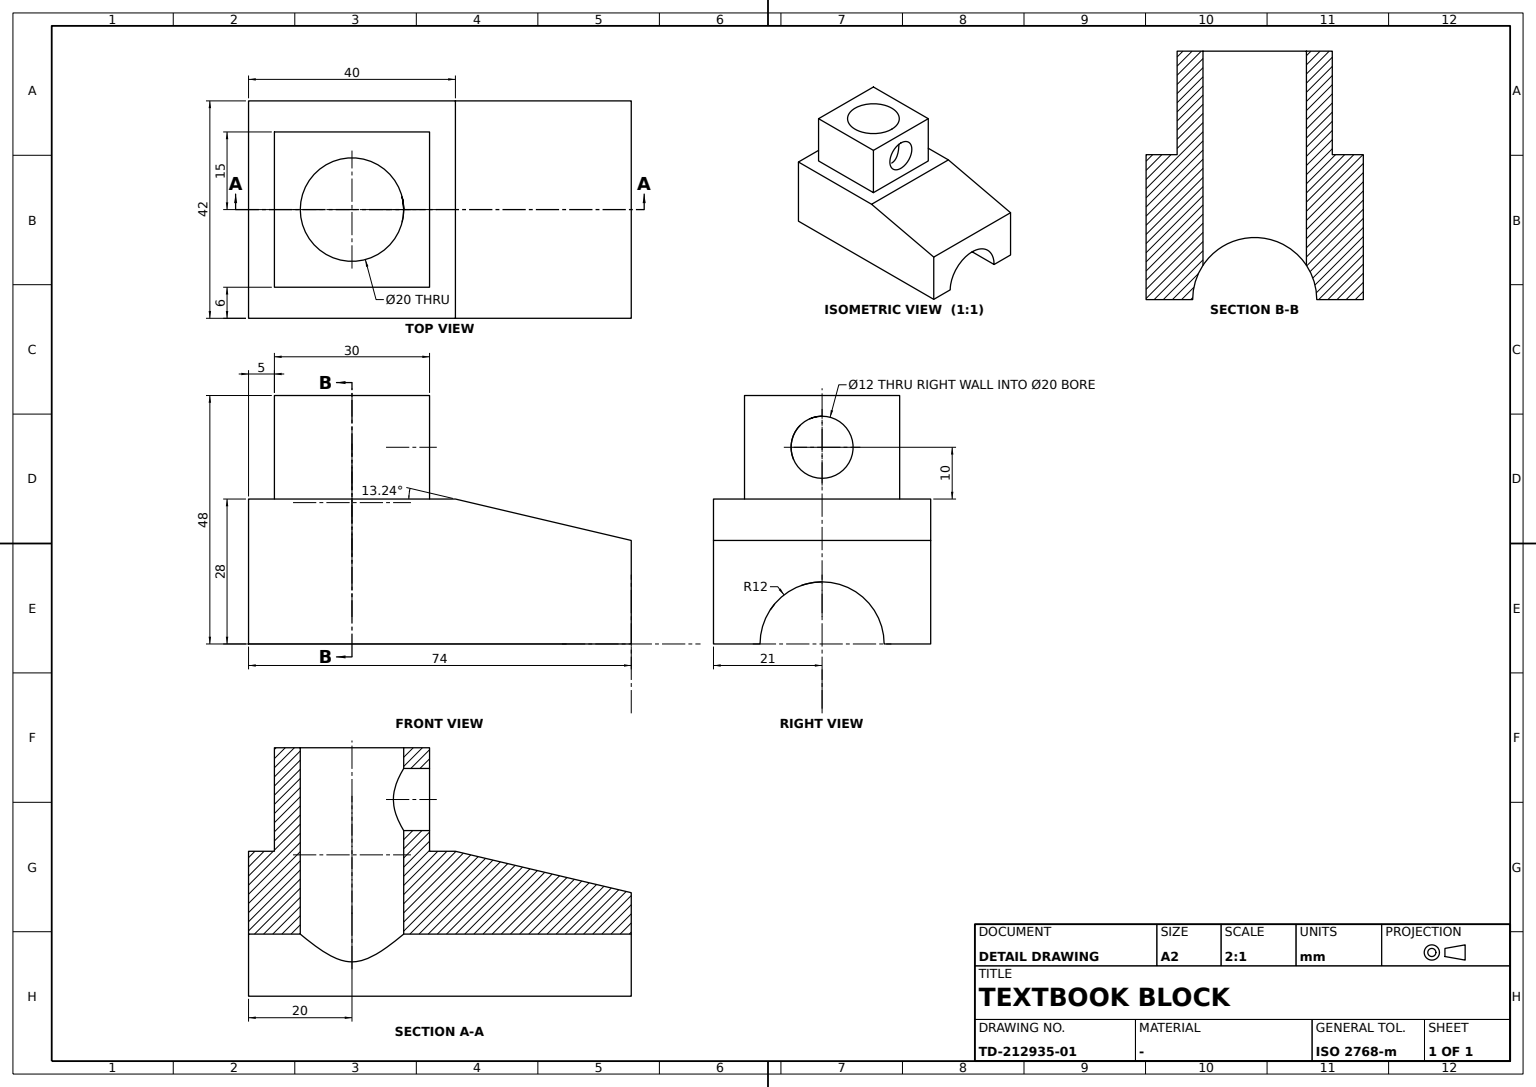
ISO-10303-21;
HEADER;
FILE_DESCRIPTION((''),'2;1');
FILE_NAME('','',(''),(''),'','','');
FILE_SCHEMA(('AUTOMOTIVE_DESIGN'));
ENDSEC;
DATA;
#1=APPLICATION_CONTEXT('');
#2=PRODUCT_CONTEXT('',#1,'mechanical');
#3=PRODUCT('','','',(#2));
#4=PRODUCT_DEFINITION_FORMATION('','',#3);
#5=PRODUCT_DEFINITION_CONTEXT('',#1,'design');
#6=PRODUCT_DEFINITION('','',#4,#5);
#7=PRODUCT_DEFINITION_SHAPE('','',#6);
#8=(LENGTH_UNIT()NAMED_UNIT(*)SI_UNIT(.MILLI.,.METRE.));
#9=(NAMED_UNIT(*)PLANE_ANGLE_UNIT()SI_UNIT($,.RADIAN.));
#10=(NAMED_UNIT(*)SI_UNIT($,.STERADIAN.)SOLID_ANGLE_UNIT());
#11=UNCERTAINTY_MEASURE_WITH_UNIT(LENGTH_MEASURE(0.005),#8,'distance_accuracy_value','');
#12=(GEOMETRIC_REPRESENTATION_CONTEXT(3)GLOBAL_UNCERTAINTY_ASSIGNED_CONTEXT((#11))GLOBAL_UNIT_ASSIGNED_CONTEXT((#8,#9,#10))REPRESENTATION_CONTEXT('',''));
#13=CARTESIAN_POINT('',(-69.,15.,48.));
#14=VERTEX_POINT('',#13);
#15=CARTESIAN_POINT('',(-39.,15.,48.));
#16=VERTEX_POINT('',#15);
#17=CARTESIAN_POINT('',(0.,15.,48.));
#18=DIRECTION('',(1.,0.,0.));
#19=VECTOR('',#18,1000.);
#20=LINE('',#17,#19);
#21=EDGE_CURVE('',#14,#16,#20,.T.);
#22=ORIENTED_EDGE('',*,*,#21,.T.);
#23=CARTESIAN_POINT('',(-39.,15.,28.));
#24=VERTEX_POINT('',#23);
#25=DIRECTION('',(0.,0.,1.));
#26=VECTOR('',#25,1000.);
#27=LINE('',#23,#26);
#28=EDGE_CURVE('',#24,#16,#27,.T.);
#29=ORIENTED_EDGE('',*,*,#28,.F.);
#30=CARTESIAN_POINT('',(-69.,15.,28.));
#31=VERTEX_POINT('',#30);
#32=CARTESIAN_POINT('',(-74.,15.,28.));
#33=LINE('',#32,#19);
#34=EDGE_CURVE('',#31,#24,#33,.T.);
#35=ORIENTED_EDGE('',*,*,#34,.F.);
#36=LINE('',#30,#26);
#37=EDGE_CURVE('',#31,#14,#36,.T.);
#38=ORIENTED_EDGE('',*,*,#37,.T.);
#39=EDGE_LOOP('',(#22,#29,#35,#38));
#40=FACE_BOUND('',#39,.T.);
#41=DIRECTION('',(0.,-1.,0.));
#42=AXIS2_PLACEMENT_3D('',#30,#41,#18);
#43=PLANE('',#42);
#44=ADVANCED_FACE('',(#40),#43,.F.);
#45=CARTESIAN_POINT('',(-39.,0.,44.));
#46=VERTEX_POINT('',#45);
#47=CARTESIAN_POINT('',(-39.,0.,38.));
#48=DIRECTION('',(-1.,0.,0.));
#49=AXIS2_PLACEMENT_3D('',#47,#48,#25);
#50=CIRCLE('',#49,6.);
#51=EDGE_CURVE('',#46,#46,#50,.F.);
#52=ORIENTED_EDGE('',*,*,#51,.T.);
#53=EDGE_LOOP('',(#52));
#54=FACE_BOUND('',#53,.T.);
#55=CARTESIAN_POINT('',(-44.,0.,44.));
#56=VERTEX_POINT('',#55);
#57=CARTESIAN_POINT('',(-45.72385,-5.648723,35.556827));
#58=CARTESIAN_POINT('',(-46.133302,-6.168929,37.968813));
#59=CARTESIAN_POINT('',(-45.742594,-5.675096,40.384956));
#60=CARTESIAN_POINT('',(-44.943937,-4.368606,42.320345));
#61=CARTESIAN_POINT('',(-44.212651,-2.441004,43.654111));
#62=CARTESIAN_POINT('',(-43.896022,-0.009852,44.168956));
#63=CARTESIAN_POINT('',(-44.203313,2.400272,43.669977));
#64=CARTESIAN_POINT('',(-44.931599,4.34478,42.344321));
#65=CARTESIAN_POINT('',(-45.726756,5.652486,40.432527));
#66=CARTESIAN_POINT('',(-46.132614,6.168125,38.027946));
#67=CARTESIAN_POINT('',(-45.74252,5.67466,35.615698));
#68=CARTESIAN_POINT('',(-44.946021,4.372806,33.684258));
#69=CARTESIAN_POINT('',(-44.215601,2.448398,32.350859));
#70=CARTESIAN_POINT('',(-43.896456,0.034977,31.831785));
#71=CARTESIAN_POINT('',(-44.198917,-2.386022,32.322571));
#72=CARTESIAN_POINT('',(-44.927018,-4.335575,33.64655));
#73=B_SPLINE_CURVE_WITH_KNOTS('',3,(#57,#58,#59,#60,#61,#62,#63,#64,#65,#66,#67,#68,#69,#70,#71,#72,#57,#58,#59),.UNSPECIFIED.,.T.,.F.,(1,1,1,1,1,1,1,1,1,1,1,1,1,1,1,1,1,1,1,1,1,1,1),(0.011996515,0.014401064,0.016805613,0.019210162,0.021614711,0.02401926,0.026423809,0.028828358,0.031232907,0.033637456,0.036042005,0.038446554,0.040851103,0.043255652,0.045660201,0.04806475,0.050469299,0.052873848,0.055278397,0.057682946,0.060087495,0.062492044,0.064896593),.UNSPECIFIED.);
#74=EDGE_CURVE('',#56,#56,#73,.T.);
#75=ORIENTED_EDGE('',*,*,#74,.T.);
#76=EDGE_LOOP('',(#75));
#77=FACE_BOUND('',#76,.T.);
#78=CARTESIAN_POINT('',(-57.16,0.,38.));
#79=DIRECTION('',(0.,1.,0.));
#80=AXIS2_PLACEMENT_3D('',#78,#18,#79);
#81=CYLINDRICAL_SURFACE('',#80,6.);
#82=ADVANCED_FACE('',(#54,#77),#81,.F.);
#83=ORIENTED_EDGE('',*,*,#74,.F.);
#84=EDGE_LOOP('',(#83));
#85=FACE_BOUND('',#84,.T.);
#86=CARTESIAN_POINT('',(-44.,0.,12.));
#87=VERTEX_POINT('',#86);
#88=CARTESIAN_POINT('',(-44.618491,-4.18439,11.477483));
#89=CARTESIAN_POINT('',(-43.691311,0.00142,12.260821));
#90=CARTESIAN_POINT('',(-44.616265,4.17871,11.479232));
#91=CARTESIAN_POINT('',(-46.872004,7.327876,9.688881));
#92=CARTESIAN_POINT('',(-49.416209,9.043886,7.953031));
#93=CARTESIAN_POINT('',(-51.902657,9.848516,6.868653));
#94=CARTESIAN_POINT('',(-53.999481,10.075679,6.515667));
#95=CARTESIAN_POINT('',(-56.095179,9.848768,6.868177));
#96=CARTESIAN_POINT('',(-58.579041,9.04633,7.95028));
#97=CARTESIAN_POINT('',(-61.128175,7.327395,9.688837));
#98=CARTESIAN_POINT('',(-63.381105,4.18509,11.477149));
#99=CARTESIAN_POINT('',(-64.308689,0.000007,12.260821));
#100=CARTESIAN_POINT('',(-63.384139,-4.178008,11.479566));
#101=CARTESIAN_POINT('',(-61.128385,-7.327527,9.689168));
#102=CARTESIAN_POINT('',(-58.584073,-9.043764,7.953186));
#103=CARTESIAN_POINT('',(-56.097488,-9.848494,6.868688));
#104=CARTESIAN_POINT('',(-54.000518,-10.07569,6.51565));
#105=CARTESIAN_POINT('',(-51.904677,-9.848746,6.868211));
#106=CARTESIAN_POINT('',(-49.420676,-9.046208,7.950437));
#107=CARTESIAN_POINT('',(-46.871436,-7.327046,9.689124));
#108=B_SPLINE_CURVE_WITH_KNOTS('',3,(#88,#89,#90,#91,#92,#93,#94,#95,#96,#97,#98,#99,#100,#101,#102,#103,#104,#105,#106,#107,#88,#89,#90),.UNSPECIFIED.,.T.,.F.,(1,1,1,1,1,1,1,1,1,1,1,1,1,1,1,1,1,1,1,1,1,1,1,1,1,1,1),(-0.012517475,-0.008344984,-0.004172492,0.,0.004172492,0.008344984,0.012517475,0.014603721,0.016689967,0.018776213,0.020862459,0.025034951,0.029207442,0.033379934,0.037552426,0.041724918,0.045897409,0.047983655,0.050069901,0.052156147,0.054242393,0.058414885,0.062587376,0.066759868,0.07093236,0.075104852,0.079277343),.UNSPECIFIED.);
#109=EDGE_CURVE('',#87,#87,#108,.T.);
#110=ORIENTED_EDGE('',*,*,#109,.F.);
#111=EDGE_LOOP('',(#110));
#112=FACE_BOUND('',#111,.T.);
#113=CARTESIAN_POINT('',(-44.,0.,48.));
#114=VERTEX_POINT('',#113);
#115=CARTESIAN_POINT('',(-54.,0.,48.));
#116=AXIS2_PLACEMENT_3D('',#115,#25,#18);
#117=CIRCLE('',#116,10.);
#118=EDGE_CURVE('',#114,#114,#117,.T.);
#119=ORIENTED_EDGE('',*,*,#118,.T.);
#120=EDGE_LOOP('',(#119));
#121=FACE_BOUND('',#120,.T.);
#122=CARTESIAN_POINT('',(-54.,0.,23.34));
#123=AXIS2_PLACEMENT_3D('',#122,#25,#18);
#124=CYLINDRICAL_SURFACE('',#123,10.);
#125=ADVANCED_FACE('',(#85,#112,#121),#124,.F.);
#126=CARTESIAN_POINT('',(-74.,-12.,0.));
#127=VERTEX_POINT('',#126);
#128=CARTESIAN_POINT('',(-74.,12.,0.));
#129=VERTEX_POINT('',#128);
#130=CARTESIAN_POINT('',(-74.,0.,0.));
#131=AXIS2_PLACEMENT_3D('',#130,#48,#25);
#132=CIRCLE('',#131,12.);
#133=EDGE_CURVE('',#127,#129,#132,.T.);
#134=ORIENTED_EDGE('',*,*,#133,.F.);
#135=CARTESIAN_POINT('',(-74.,-21.,0.));
#136=VERTEX_POINT('',#135);
#137=VECTOR('',#79,1000.);
#138=LINE('',#130,#137);
#139=EDGE_CURVE('',#136,#127,#138,.T.);
#140=ORIENTED_EDGE('',*,*,#139,.F.);
#141=CARTESIAN_POINT('',(-74.,-21.,28.));
#142=VERTEX_POINT('',#141);
#143=LINE('',#135,#26);
#144=EDGE_CURVE('',#136,#142,#143,.T.);
#145=ORIENTED_EDGE('',*,*,#144,.T.);
#146=CARTESIAN_POINT('',(-74.,21.,28.));
#147=VERTEX_POINT('',#146);
#148=CARTESIAN_POINT('',(-74.,0.,28.));
#149=LINE('',#148,#137);
#150=EDGE_CURVE('',#142,#147,#149,.T.);
#151=ORIENTED_EDGE('',*,*,#150,.T.);
#152=CARTESIAN_POINT('',(-74.,21.,0.));
#153=VERTEX_POINT('',#152);
#154=LINE('',#152,#26);
#155=EDGE_CURVE('',#153,#147,#154,.T.);
#156=ORIENTED_EDGE('',*,*,#155,.F.);
#157=EDGE_CURVE('',#129,#153,#138,.T.);
#158=ORIENTED_EDGE('',*,*,#157,.F.);
#159=EDGE_LOOP('',(#134,#140,#145,#151,#156,#158));
#160=FACE_BOUND('',#159,.T.);
#161=PLANE('',#131);
#162=ADVANCED_FACE('',(#160),#161,.T.);
#163=CARTESIAN_POINT('',(0.,21.,20.));
#164=VERTEX_POINT('',#163);
#165=CARTESIAN_POINT('',(0.,21.,0.));
#166=VERTEX_POINT('',#165);
#167=DIRECTION('',(0.,0.,-1.));
#168=VECTOR('',#167,1000.);
#169=LINE('',#165,#168);
#170=EDGE_CURVE('',#164,#166,#169,.T.);
#171=ORIENTED_EDGE('',*,*,#170,.T.);
#172=VECTOR('',#48,1000.);
#173=LINE('',#165,#172);
#174=EDGE_CURVE('',#166,#153,#173,.T.);
#175=ORIENTED_EDGE('',*,*,#174,.T.);
#176=ORIENTED_EDGE('',*,*,#155,.T.);
#177=CARTESIAN_POINT('',(-34.,21.,28.));
#178=VERTEX_POINT('',#177);
#179=CARTESIAN_POINT('',(0.,21.,28.));
#180=LINE('',#179,#19);
#181=EDGE_CURVE('',#147,#178,#180,.T.);
#182=ORIENTED_EDGE('',*,*,#181,.T.);
#183=CARTESIAN_POINT('',(4.459016,21.,18.95082));
#184=DIRECTION('',(0.973417168,0.,-0.229039334));
#185=VECTOR('',#184,1000.);
#186=LINE('',#183,#185);
#187=EDGE_CURVE('',#178,#164,#186,.T.);
#188=ORIENTED_EDGE('',*,*,#187,.T.);
#189=EDGE_LOOP('',(#171,#175,#176,#182,#188));
#190=FACE_BOUND('',#189,.T.);
#191=AXIS2_PLACEMENT_3D('',#165,#79,#48);
#192=PLANE('',#191);
#193=ADVANCED_FACE('',(#190),#192,.T.);
#194=CARTESIAN_POINT('',(-69.,-15.,48.));
#195=VERTEX_POINT('',#194);
#196=CARTESIAN_POINT('',(-69.,0.,48.));
#197=LINE('',#196,#137);
#198=EDGE_CURVE('',#195,#14,#197,.T.);
#199=ORIENTED_EDGE('',*,*,#198,.F.);
#200=CARTESIAN_POINT('',(-39.,-15.,48.));
#201=VERTEX_POINT('',#200);
#202=CARTESIAN_POINT('',(0.,-15.,48.));
#203=LINE('',#202,#172);
#204=EDGE_CURVE('',#201,#195,#203,.T.);
#205=ORIENTED_EDGE('',*,*,#204,.F.);
#206=CARTESIAN_POINT('',(-39.,0.,48.));
#207=VECTOR('',#41,1000.);
#208=LINE('',#206,#207);
#209=EDGE_CURVE('',#16,#201,#208,.T.);
#210=ORIENTED_EDGE('',*,*,#209,.F.);
#211=ORIENTED_EDGE('',*,*,#21,.F.);
#212=EDGE_LOOP('',(#199,#205,#210,#211));
#213=FACE_BOUND('',#212,.T.);
#214=ORIENTED_EDGE('',*,*,#118,.F.);
#215=EDGE_LOOP('',(#214));
#216=FACE_BOUND('',#215,.T.);
#217=CARTESIAN_POINT('',(0.,0.,48.));
#218=AXIS2_PLACEMENT_3D('',#217,#25,#18);
#219=PLANE('',#218);
#220=ADVANCED_FACE('',(#213,#216),#219,.T.);
#221=ORIENTED_EDGE('',*,*,#174,.F.);
#222=CARTESIAN_POINT('',(0.,12.,0.));
#223=VERTEX_POINT('',#222);
#224=CARTESIAN_POINT('',(0.,0.,0.));
#225=LINE('',#224,#137);
#226=EDGE_CURVE('',#223,#166,#225,.T.);
#227=ORIENTED_EDGE('',*,*,#226,.F.);
#228=LINE('',#128,#19);
#229=EDGE_CURVE('',#223,#129,#228,.F.);
#230=ORIENTED_EDGE('',*,*,#229,.T.);
#231=ORIENTED_EDGE('',*,*,#157,.T.);
#232=EDGE_LOOP('',(#221,#227,#230,#231));
#233=FACE_BOUND('',#232,.T.);
#234=AXIS2_PLACEMENT_3D('',#224,#167,#48);
#235=PLANE('',#234);
#236=ADVANCED_FACE('',(#233),#235,.T.);
#237=CARTESIAN_POINT('',(0.,-21.,0.));
#238=VERTEX_POINT('',#237);
#239=LINE('',#237,#172);
#240=EDGE_CURVE('',#238,#136,#239,.T.);
#241=ORIENTED_EDGE('',*,*,#240,.T.);
#242=ORIENTED_EDGE('',*,*,#139,.T.);
#243=CARTESIAN_POINT('',(0.,-12.,0.));
#244=VERTEX_POINT('',#243);
#245=LINE('',#126,#19);
#246=EDGE_CURVE('',#127,#244,#245,.T.);
#247=ORIENTED_EDGE('',*,*,#246,.T.);
#248=EDGE_CURVE('',#238,#244,#225,.T.);
#249=ORIENTED_EDGE('',*,*,#248,.F.);
#250=EDGE_LOOP('',(#241,#242,#247,#249));
#251=FACE_BOUND('',#250,.T.);
#252=ADVANCED_FACE('',(#251),#235,.T.);
#253=CARTESIAN_POINT('',(-34.,-21.,28.));
#254=VERTEX_POINT('',#253);
#255=CARTESIAN_POINT('',(0.,-21.,20.));
#256=VERTEX_POINT('',#255);
#257=CARTESIAN_POINT('',(4.459016,-21.,18.95082));
#258=LINE('',#257,#185);
#259=EDGE_CURVE('',#254,#256,#258,.T.);
#260=ORIENTED_EDGE('',*,*,#259,.T.);
#261=CARTESIAN_POINT('',(0.,0.,20.));
#262=LINE('',#261,#137);
#263=EDGE_CURVE('',#256,#164,#262,.T.);
#264=ORIENTED_EDGE('',*,*,#263,.T.);
#265=ORIENTED_EDGE('',*,*,#187,.F.);
#266=CARTESIAN_POINT('',(-34.,0.,28.));
#267=LINE('',#266,#137);
#268=EDGE_CURVE('',#254,#178,#267,.T.);
#269=ORIENTED_EDGE('',*,*,#268,.F.);
#270=EDGE_LOOP('',(#260,#264,#265,#269));
#271=FACE_BOUND('',#270,.T.);
#272=DIRECTION('',(0.229039334,0.,0.973417168));
#273=AXIS2_PLACEMENT_3D('',#266,#272,#184);
#274=PLANE('',#273);
#275=ADVANCED_FACE('',(#271),#274,.T.);
#276=ORIENTED_EDGE('',*,*,#34,.T.);
#277=CARTESIAN_POINT('',(-39.,-15.,28.));
#278=VERTEX_POINT('',#277);
#279=CARTESIAN_POINT('',(-39.,0.,28.));
#280=LINE('',#279,#207);
#281=EDGE_CURVE('',#24,#278,#280,.T.);
#282=ORIENTED_EDGE('',*,*,#281,.T.);
#283=CARTESIAN_POINT('',(-69.,-15.,28.));
#284=VERTEX_POINT('',#283);
#285=CARTESIAN_POINT('',(-74.,-15.,28.));
#286=LINE('',#285,#172);
#287=EDGE_CURVE('',#278,#284,#286,.T.);
#288=ORIENTED_EDGE('',*,*,#287,.T.);
#289=CARTESIAN_POINT('',(-69.,0.,28.));
#290=LINE('',#289,#137);
#291=EDGE_CURVE('',#284,#31,#290,.T.);
#292=ORIENTED_EDGE('',*,*,#291,.T.);
#293=EDGE_LOOP('',(#276,#282,#288,#292));
#294=FACE_BOUND('',#293,.T.);
#295=ORIENTED_EDGE('',*,*,#181,.F.);
#296=ORIENTED_EDGE('',*,*,#150,.F.);
#297=CARTESIAN_POINT('',(0.,-21.,28.));
#298=LINE('',#297,#19);
#299=EDGE_CURVE('',#142,#254,#298,.T.);
#300=ORIENTED_EDGE('',*,*,#299,.T.);
#301=ORIENTED_EDGE('',*,*,#268,.T.);
#302=EDGE_LOOP('',(#295,#296,#300,#301));
#303=FACE_BOUND('',#302,.T.);
#304=AXIS2_PLACEMENT_3D('',#148,#25,#18);
#305=PLANE('',#304);
#306=ADVANCED_FACE('',(#294,#303),#305,.T.);
#307=ORIENTED_EDGE('',*,*,#291,.F.);
#308=LINE('',#283,#26);
#309=EDGE_CURVE('',#284,#195,#308,.T.);
#310=ORIENTED_EDGE('',*,*,#309,.T.);
#311=ORIENTED_EDGE('',*,*,#198,.T.);
#312=ORIENTED_EDGE('',*,*,#37,.F.);
#313=EDGE_LOOP('',(#307,#310,#311,#312));
#314=FACE_BOUND('',#313,.T.);
#315=AXIS2_PLACEMENT_3D('',#283,#18,#79);
#316=PLANE('',#315);
#317=ADVANCED_FACE('',(#314),#316,.F.);
#318=ORIENTED_EDGE('',*,*,#259,.F.);
#319=ORIENTED_EDGE('',*,*,#299,.F.);
#320=ORIENTED_EDGE('',*,*,#144,.F.);
#321=ORIENTED_EDGE('',*,*,#240,.F.);
#322=LINE('',#237,#168);
#323=EDGE_CURVE('',#256,#238,#322,.T.);
#324=ORIENTED_EDGE('',*,*,#323,.F.);
#325=EDGE_LOOP('',(#318,#319,#320,#321,#324));
#326=FACE_BOUND('',#325,.T.);
#327=AXIS2_PLACEMENT_3D('',#237,#79,#48);
#328=PLANE('',#327);
#329=ADVANCED_FACE('',(#326),#328,.F.);
#330=ORIENTED_EDGE('',*,*,#204,.T.);
#331=ORIENTED_EDGE('',*,*,#309,.F.);
#332=ORIENTED_EDGE('',*,*,#287,.F.);
#333=LINE('',#277,#26);
#334=EDGE_CURVE('',#278,#201,#333,.T.);
#335=ORIENTED_EDGE('',*,*,#334,.T.);
#336=EDGE_LOOP('',(#330,#331,#332,#335));
#337=FACE_BOUND('',#336,.T.);
#338=AXIS2_PLACEMENT_3D('',#277,#79,#48);
#339=PLANE('',#338);
#340=ADVANCED_FACE('',(#337),#339,.F.);
#341=ORIENTED_EDGE('',*,*,#246,.F.);
#342=ORIENTED_EDGE('',*,*,#133,.T.);
#343=ORIENTED_EDGE('',*,*,#229,.F.);
#344=AXIS2_PLACEMENT_3D('',#224,#18,#167);
#345=CIRCLE('',#344,12.);
#346=EDGE_CURVE('',#223,#244,#345,.T.);
#347=ORIENTED_EDGE('',*,*,#346,.T.);
#348=EDGE_LOOP('',(#341,#342,#343,#347));
#349=FACE_BOUND('',#348,.T.);
#350=ORIENTED_EDGE('',*,*,#109,.T.);
#351=EDGE_LOOP('',(#350));
#352=FACE_BOUND('',#351,.T.);
#353=CARTESIAN_POINT('',(-37.66,0.,0.));
#354=AXIS2_PLACEMENT_3D('',#353,#18,#79);
#355=CYLINDRICAL_SURFACE('',#354,12.);
#356=ADVANCED_FACE('',(#349,#352),#355,.F.);
#357=ORIENTED_EDGE('',*,*,#226,.T.);
#358=ORIENTED_EDGE('',*,*,#170,.F.);
#359=ORIENTED_EDGE('',*,*,#263,.F.);
#360=ORIENTED_EDGE('',*,*,#323,.T.);
#361=ORIENTED_EDGE('',*,*,#248,.T.);
#362=ORIENTED_EDGE('',*,*,#346,.F.);
#363=EDGE_LOOP('',(#357,#358,#359,#360,#361,#362));
#364=FACE_BOUND('',#363,.T.);
#365=AXIS2_PLACEMENT_3D('',#261,#18,#167);
#366=PLANE('',#365);
#367=ADVANCED_FACE('',(#364),#366,.T.);
#368=ORIENTED_EDGE('',*,*,#209,.T.);
#369=ORIENTED_EDGE('',*,*,#334,.F.);
#370=ORIENTED_EDGE('',*,*,#281,.F.);
#371=ORIENTED_EDGE('',*,*,#28,.T.);
#372=EDGE_LOOP('',(#368,#369,#370,#371));
#373=FACE_BOUND('',#372,.T.);
#374=ORIENTED_EDGE('',*,*,#51,.F.);
#375=EDGE_LOOP('',(#374));
#376=FACE_BOUND('',#375,.T.);
#377=AXIS2_PLACEMENT_3D('',#23,#48,#41);
#378=PLANE('',#377);
#379=ADVANCED_FACE('',(#373,#376),#378,.F.);
#380=CLOSED_SHELL('',(#44,#82,#125,#162,#193,#220,#236,#252,#275,#306,#317,#329,#340,#356,#367,#379));
#381=MANIFOLD_SOLID_BREP('',#380);
#382=ADVANCED_BREP_SHAPE_REPRESENTATION('',(#381),#12);
#383=SHAPE_DEFINITION_REPRESENTATION(#7,#382);
ENDSEC;
END-ISO-10303-21;
